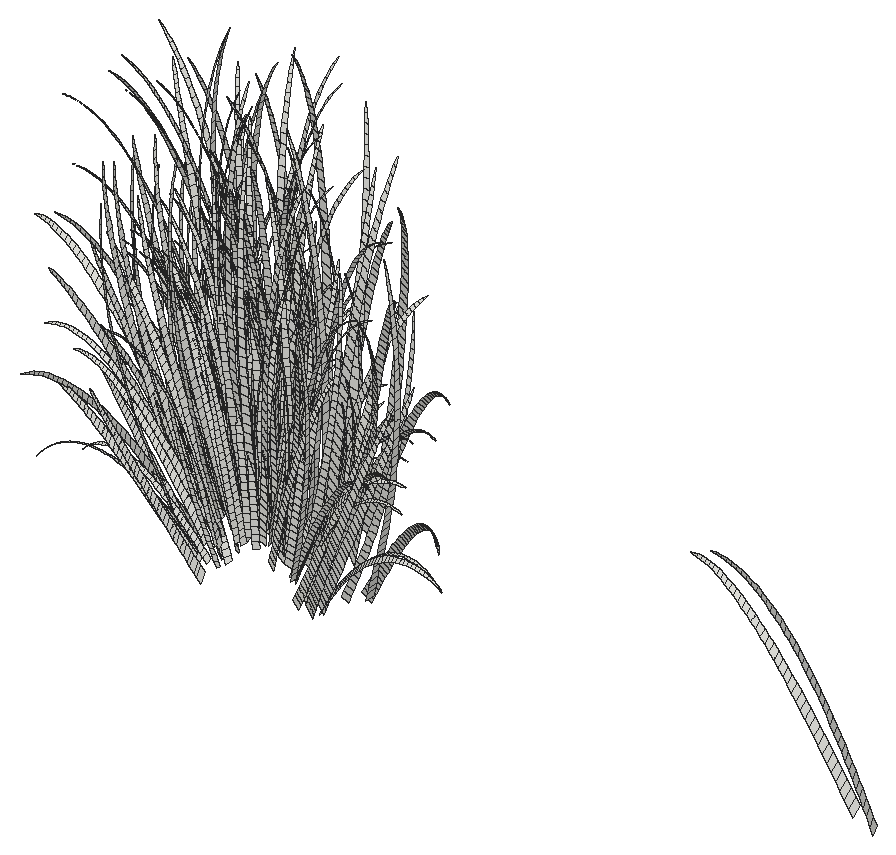
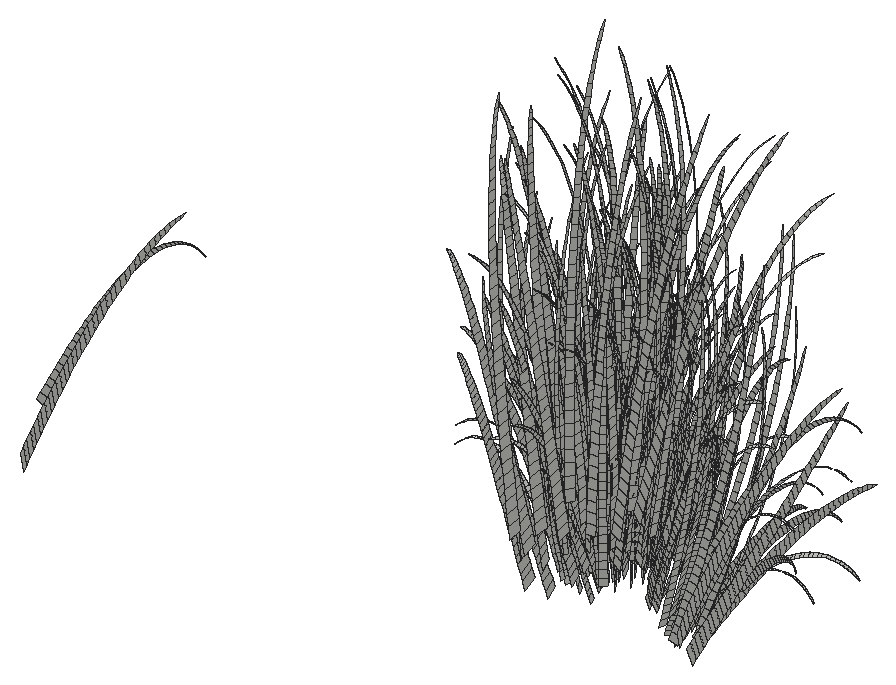
# SketchUp Ruby script. Lengths in inches.
U = 1.inch
M = Sketchup.active_model
def pt(a) = Geom::Point3d.new(a.map { |v| v * U })
def face(e, loops, mat)
  f = e.add_face(loops[0].map { |a| pt(a) })
  loops[1..].each { |l| e.add_face(l.map { |a| pt(a) }).erase! }
  f.material = f.back_material = mat if mat
  f
end
# faces: each face lists its corners as indices into pts; further lists are holes
def faces(e, pts, list, mat = nil) = list.each { |f| face(e, (f[0].is_a?(Array) ? f : [f]).map { |l| l.map { |i| pts[i] } }, mat) }
# xy, xz, yz: faces in a plane at the given z, y or x. An outline is a flat list of corners, or four numbers for a rectangle; further outlines are holes
def ring(l) = l.size == 4 ? [[l[0], l[1]], [l[2], l[1]], [l[2], l[3]], [l[0], l[3]]] : l.each_slice(2).to_a
def flat(e, list, mat, &to3) = list.each { |f| face(e, (f[0].is_a?(Array) ? f : [f]).map { |l| ring(l).map { |u, v| to3.(u, v) } }, mat) }
def xy(e, z, list, mat = nil) = flat(e, list, mat) { |x, y| [x, y, z] }
def xz(e, y, list, mat = nil) = flat(e, list, mat) { |x, z| [x, y, z] }
def yz(e, x, list, mat = nil) = flat(e, list, mat) { |y, z| [x, y, z] }
def lines(e, pts, list) = list.each { |a, b| e.add_line(pt(pts[a]), pt(pts[b])) }
# prism: a flat outline (further loops are holes) pulled along v
def prism(e, loops, v, mat = nil)
  f = face(e, loops, mat); d = Geom::Vector3d.new(v.map { |x| x * U })
  f.pushpull(f.normal.samedirection?(d) ? d.length : -d.length)
end
def box(e, o, s, mat = nil) = prism(e, [[o, [o[0] + s[0], o[1], o[2]], [o[0] + s[0], o[1] + s[1], o[2]], [o[0], o[1] + s[1], o[2]]]], [0, 0, s[2]], mat)
def at(x, y, z, deg = 0) = Geom::Transformation.translation(pt([x, y, z])) * Geom::Transformation.rotation(ORIGIN, Z_AXIS, deg.degrees)
def axes(o, x, y, z) = Geom::Transformation.new([*x, 0, *y, 0, *z, 0, *pt(o).to_a, 1])
def part(name) = M.definitions.add(name)
# library, detail: a bought-in or finely detailed component or shape, given as its bounding box
def library(name, o, s) = part(name).tap { |d| box(d.entities, o, s) }
def detail(e, o, s) = box(e.add_group.entities, o, s)
def put(e, d, t, mat = nil) = e.add_instance(d, t).tap { |i| i.material = mat if mat }
def group(e, t, mat = nil) = e.add_group.tap { |g| g.transformation = t; g.material = mat if mat }.entities
root = M.entities
c1 = part("fur_instance\#8")
p = [[-0.25,1.49,0.03],[0.25,-1.49,-0.03],[0.44,-1.47,1.51],[-0.05,1.47,1.57],[0.65,-1.44,3.05],[0.16,1.45,3.11],
  [0.86,-1.42,4.59],[0.38,1.44,4.65],[1.1,-1.39,6.13],[0.62,1.43,6.18],[1.34,-1.35,7.66],[0.875,1.42,7.72],
  [1.6,-1.32,9.19],[1.14,1.41,9.25],[1.88,-1.28,10.72],[1.43,1.41,10.78],[2.18,-1.24,12.25],[1.73,1.41,12.3],
  [2.49,-1.19,13.77],[2.05,1.41,13.82],[2.83,-1.15,15.29],[2.4,1.41,15.34],[3.18,-1.09,16.8],[2.76,1.42,16.85],
  [3.56,-1.03,18.31],[3.14,1.43,18.35],[3.96,-0.97,19.81],[3.55,1.44,19.85],[4.38,-0.91,21.3],[3.99,1.46,21.35],
  [4.84,-0.83,22.78],[4.45,1.48,22.83],[5.32,-0.76,24.26],[4.93,1.51,24.31],[5.82,-0.67,25.73],[5.45,1.54,25.77],
  [6.36,-0.59,27.18],[6,1.57,27.23],[6.93,-0.49,28.625],[6.58,1.61,28.67],[7.54,-0.39,30.05],[7.19,1.66,30.1],
  [8.18,-0.28,31.47],[7.84,1.71,31.51],[8.85,-0.16,32.86],[8.53,1.77,32.9],[9.57,-0.04,34.24],[9.25,1.83,34.27],
  [10.32,0.09,35.59],[10.02,1.9,35.625],[11.12,0.23,36.92],[10.82,1.97,36.95],[11.95,0.38,38.22],[11.67,2.06,38.25],
  [12.84,0.54,39.49],[12.57,2.14,39.52],[13.76,0.71,40.73],[13.51,2.24,40.76],[14.73,0.89,41.93],[14.49,2.34,41.95],
  [15.75,1.08,43.09],[15.52,2.45,43.11],[16.82,1.28,44.2],[16.6,2.5625,44.23],[17.93,1.5,45.27],[17.73,2.68,45.29],
  [19.08,1.73,46.28],[18.9,2.81,46.3],[20.29,1.97,47.24],[20.125,2.93,47.26],[21.53,2.22,48.13],[21.39,3.0625,48.15],
  [22.82,2.5,48.96],[22.7,3.1875,48.98],[24.14,2.8125,49.72],[24.06,3.3,49.73],[25.48,3.27,50.41]]
faces(c1.entities,p,[[0,1,2,3],[3,2,4,5],[5,4,6,7],[7,6,8,9],[9,8,10,11],[11,10,12,13],[13,12,14,15],[15,14,16,17],
  [17,16,18,19],[19,18,20,21],[21,20,22,23],[23,22,24,25],[25,24,26,27],[27,26,28,29],[29,28,30,31],[31,30,32,33],
  [33,32,34,35],[35,34,36,37],[37,36,38,39],[39,38,40,41],[41,40,42,43],[43,42,44,45],[45,44,46,47],[47,46,48,49],
  [49,48,50,51],[51,50,52,53],[53,52,54,55],[55,54,56,57],[57,56,58,59],[59,58,60,61],[61,60,62,63],[63,62,64,65],
  [65,64,66,67],[67,66,68,69],[69,68,70,71],[71,70,72,73],[73,72,74,75],[75,74,76]])
put(root,c1,axes([43.23,68.45,7.65],[-0.18691,0.1568,-0.23935],[-0.06787,-0.16218,-0.27405],[-0.15492,-0.08418,0.43132]))
put(root,c1,axes([42.47,71.27,4.78],[-0.09014,-0.18111,-0.08882],[0.15594,-0.13199,0.32093],[-0.15035,0.00199,0.40617]))
put(root,c1,axes([42.5,70.05,2.88],[0.01897,-0.21218,0.0586],[0.13531,-0.01729,0.38322],[-0.17657,-0.01268,0.31544]))
put(root,c1,axes([43.08,68.3125,3.14],[-0.03242,-0.16161,-0.19656],[0.13271,-0.12456,0.32589],[-0.17032,-0.04313,0.30667]))
put(root,c1,axes([44.46,67.32,5.39],[-0.17146,0.07712,-0.27655],[0.00216,-0.17859,-0.14821],[-0.13359,-0.07259,0.37194]))
put(root,c1,axes([44.12,67.44,2.26],[-0.07927,0.1771,-0.13212],[-0.09456,-0.05104,-0.31736],[-0.15384,-0.03896,0.27701]))
put(root,c1,axes([44.33,67.0625,3.02],[-0.11039,-0.00414,-0.3495],[0.07669,-0.1786,0.00651],[-0.14786,-0.06719,0.2791]))
put(root,c1,axes([44.91,65.8125,3.03],[-0.13594,0.15084,-0.11164],[-0.0609,-0.07291,-0.33491],[-0.13519,-0.09407,0.27953]))
put(root,c1,axes([42.62,69.58,3.24],[0.13391,-0.00422,0.37894],[-0.02725,0.21287,-0.08205],[-0.17659,-0.01268,0.31548]))
put(root,c1,axes([45.3,66.53,4.31],[-0.14992,0.10635,-0.20855],[-0.03569,-0.13875,-0.18978],[-0.12006,-0.06524,0.33426]))
put(root,c1,axes([45.29,67.96,4.18],[-0.13947,0.07457,-0.26376],[-0.03048,-0.16347,-0.05841],[-0.12421,-0.01975,0.3263]))
put(root,c1,axes([45.33,66.7,2.78],[-0.11214,0.07357,-0.29467],[-0.00419,-0.1506,-0.10442],[-0.13991,-0.03543,0.25192]))
put(root,c1,axes([44.39,70.26,10.76],[-0.16722,-0.14584,-0.14657],[0.18274,-0.19209,0.09427],[-0.0816,-0.06233,0.55718]))
put(root,c1,axes([42.92,71.21,4.29],[0.10956,-0.18152,0.25882],[0.13509,0.11782,0.19082],[-0.14519,0.00192,0.39222]))
put(root,c1,axes([43.91,69.17,3.66],[0.07012,-0.18381,0.20265],[0.10518,0.07075,0.29594],[-0.16336,-0.01173,0.29184]))
put(root,c1,axes([43.8,66.95,3.01],[0.11177,0.01694,0.37048],[-0.08915,0.18926,-0.03147],[-0.15727,-0.07147,0.29687]))
put(root,c1,axes([44.32,67.58,3.52],[0.07273,0.09595,0.27862],[-0.10249,0.16133,-0.212],[-0.15668,-0.03967,0.28211]))
put(root,c1,axes([42.84,68.47,4.28],[0.16226,-0.13696,0.26442],[0.06401,0.16282,0.19515],[-0.14822,-0.05035,0.39313]))
put(root,c1,axes([45.68,68.57,9.3],[-0.19486,-0.07064,-0.15993],[0.11436,-0.20339,0.01183],[-0.07048,-0.06892,0.50496]))
put(root,c1,axes([45.89,65.35,2.36],[-0.09839,0.14314,-0.01192],[-0.08354,-0.02419,-0.30566],[-0.11714,-0.08151,0.24221]))
put(root,c1,axes([45.28,68.2,2.86],[-0.01321,-0.17005,0.06481],[0.1141,-0.02557,0.30569],[-0.13946,0.01456,0.25678]))
put(root,c1,axes([46.39,69.16,7.12],[-0.18243,0.01895,-0.19563],[-0.00133,-0.1948,0.08688],[-0.09334,0.00298,0.40574]))
put(root,c1,axes([46.26,67.88,5.17],[-0.16023,0.03354,-0.19126],[-0.00898,-0.17162,0.02853],[-0.08895,-0.01176,0.36236]))
put(root,c1,axes([46.22,66.625,6.5],[-0.1494,0.14445,-0.05993],[-0.10862,-0.10225,-0.21391],[-0.08642,-0.08137,0.39881]))
put(root,c1,axes([43.7,68.125,5.17],[0.16036,-0.12824,0.26431],[0.05712,0.1633,0.18167],[-0.14465,-0.04914,0.38366]))
put(root,c1,axes([44.12,68.18,4.39],[0.12489,0.06673,0.27563],[-0.09958,0.18305,-0.12082],[-0.13573,-0.04611,0.36]))
put(root,c1,axes([46.51,66.73,5.01],[-0.15052,-0.00251,-0.18515],[0.03159,-0.16716,0.03488],[-0.08794,-0.02622,0.34898]))
put(root,c1,axes([46.24,68.69,5.72],[-0.10618,-0.13262,-0.04878],[0.13367,-0.1263,0.19427],[-0.08735,0.00279,0.37967]))
put(root,c1,axes([45.09,68.18,2.35],[0.10833,0.05099,0.24664],[-0.03776,0.16401,-0.19126],[-0.1393,0.01454,0.25647]))
put(root,c1,axes([46.21,70.78,11.94],[-0.09372,-0.20637,-0.07363],[0.22677,-0.12712,0.15354],[-0.08199,-0.04812,0.55353]))
put(root,c1,axes([44.63,69.19,4.82],[0.15491,-0.05585,0.29054],[0.02871,0.18789,-0.02061],[-0.13151,0.00174,0.35528]))
put(root,c1,axes([47.24,67.92,6.26],[-0.13836,0.10656,-0.19014],[-0.08729,-0.13946,-0.02631],[-0.08371,0.00267,0.36384]))
put(root,c1,axes([46.12,66.87,4.0625],[0.03066,0.14936,0.05869],[-0.12804,0.07175,-0.24213],[-0.11455,-0.01821,0.30092]))
put(root,c1,axes([46.49,66.9375,7.95],[-0.03053,0.18634,0.11663],[-0.19498,0.03215,-0.20672],[-0.09234,-0.08694,0.42611]))
put(root,c1,axes([46.73,66.09,6.54],[-0.076,0.1669,0.09562],[-0.17144,-0.01335,-0.19918],[-0.07397,-0.09509,0.39348]))
put(root,c1,axes([47.05,67.9,6.875],[-0.14595,-0.08896,-0.08701],[0.11069,-0.159,0.08949],[-0.05969,-0.02587,0.41282]))
put(root,c1,axes([47.0625,66.87,7.05],[-0.13003,0.1505,-0.04051],[-0.13515,-0.09639,-0.12681],[-0.0585,-0.05721,0.41915]))
put(root,c1,axes([47.05,69.73,10.85],[-0.20007,-0.1011,-0.05198],[0.13259,-0.20105,0.02025],[-0.03025,-0.05245,0.53866]))
put(root,c1,axes([47.55,69.61,11.96],[-0.23914,-0.05106,-0.06078],[0.08551,-0.22855,-0.0252],[-0.02809,-0.06875,0.5682]))
put(root,c1,axes([45.99,67.93,2.35],[0.06974,-0.11239,0.27242],[0.09117,0.10684,0.0892],[-0.12045,0.03482,0.23783]))
put(root,c1,axes([45.17,69.49,3.94],[0.12819,-0.10555,0.27193],[0.08655,0.15023,0.02614],[-0.11644,0.02211,0.33646]))
put(root,c1,axes([46.16,66.64,2.65],[0.09888,-0.02928,0.28041],[-0.00291,0.15131,-0.01175],[-0.12783,-0.00918,0.22836]))
put(root,c1,axes([46.68,68.41,4.28],[-0.01787,-0.16163,0.13786],[0.14541,-0.01364,0.20157],[-0.09392,0.03632,0.30351]))
put(root,c1,axes([47.6,66.9,6.07],[-0.15295,0.08658,-0.10984],[-0.06653,-0.14152,-0.02919],[-0.05435,-0.02356,0.3759]))
put(root,c1,axes([47.26,68.36,4.31],[-0.08732,-0.12975,0.07004],[0.12156,-0.08169,0.22443],[-0.07712,0.04857,0.29461]))
put(root,c1,axes([48.08,69.47,12.02],[-0.24023,0.10194,-0.01182],[-0.08393,-0.20819,-0.06775],[-0.02132,-0.07588,0.56748]))
put(root,c1,axes([45.8,66.95,4],[0.13512,-0.04534,0.25565],[0.00767,0.16418,0.01521],[-0.11775,-0.01872,0.30933]))
put(root,c1,axes([47.95,66.88,6.03],[-0.16155,0.04363,-0.11105],[-0.02173,-0.15615,0.00187],[-0.05311,-0.02302,0.36735]))
put(root,c1,axes([47.87,68.14,5.93],[-0.13763,-0.08778,-0.02445],[0.09224,-0.14199,0.18002],[-0.06167,0.02548,0.35158]))
put(root,c1,axes([47.56,67.91,10.37],[-0.11071,0.19643,0.08485],[-0.20741,-0.05916,-0.14436],[-0.04649,-0.10158,0.50968]))
put(root,c1,axes([45.88,67.375,6.29],[0.12398,0.09622,0.18511],[-0.12468,0.16008,-0.11198],[-0.09878,-0.04719,0.39625]))
put(root,c1,axes([48.19,67.29,6.85],[-0.15275,-0.06369,-0.07605],[0.08272,-0.1606,0.08732],[-0.05298,-0.01559,0.38969]))
put(root,c1,axes([48.03,66.44,6.02],[-0.12167,0.12231,-0.08026],[-0.10576,-0.10199,-0.07795],[-0.05387,-0.03162,0.36369]))
put(root,c1,axes([46.53,67.73,6.44],[0.1073,0.11537,0.13468],[-0.12896,0.14123,-0.15523],[-0.09593,-0.0286,0.38067]))
put(root,c1,axes([48.43,66.98,5.86],[-0.15222,0.06371,-0.10078],[-0.04912,-0.14483,0.02613],[-0.04368,-0.00705,0.35627]))
put(root,c1,axes([48.58,66.57,7.68],[-0.18454,0.07316,-0.01839],[-0.05778,-0.16138,-0.04792],[-0.01906,-0.05522,0.43193]))
put(root,c1,axes([47.28,71.5625,10.61],[-0.03022,-0.22611,0.09029],[0.23429,-0.05028,0.11994],[-0.05481,-0.00145,0.5217]))
put(root,c1,axes([46.77,65.9,6.75],[0.08886,0.11953,0.22309],[-0.17307,0.12603,-0.0526],[-0.07674,-0.09865,0.40821]))
put(root,c1,axes([48.6875,69.69,11.16],[-0.19122,-0.11806,-0.01455],[0.14538,-0.19433,0.04316],[-0.02276,-0.03764,0.53822]))
put(root,c1,axes([47.69,68.76,7.33],[-0.07059,-0.16734,0.04684],[0.17777,-0.08469,0.11217],[-0.04438,-0.00118,0.42241]))
put(root,c1,axes([48.78,67.4,6.72],[-0.1632,-0.04584,-0.02491],[0.06111,-0.16287,0.10545],[-0.03205,0.00396,0.38155]))
put(root,c1,axes([48.01,67.78,6.35],[-0.07809,-0.14325,0.0107],[0.15359,-0.09235,0.11164],[-0.04706,-0.00759,0.38378]))
put(root,c1,axes([48.86,68.24,7.62],[-0.18597,0.0618,-0.02273],[-0.04748,-0.17087,0.02426],[-0.01189,-0.02692,0.4292]))
put(root,c1,axes([47.125,67.35,3.82],[0.12505,0.02128,0.17693],[-0.02026,0.14885,-0.13694],[-0.09536,0.01811,0.27556]))
put(root,c1,axes([45.24,70.37,10.84],[0.23978,-0.07082,0.15768],[0.03022,0.22441,0.06362],[-0.07961,-0.06081,0.54364]))
put(root,c1,axes([47.99,68.31,8.97],[-0.04674,0.1979,-0.00041],[-0.20698,-0.02041,-0.04932],[-0.02674,-0.04637,0.47621]))
put(root,c1,axes([45.64,68.09,10.33],[0.21026,0.07749,0.17035],[-0.13208,0.20951,0.0486],[-0.06062,-0.09852,0.54406]))
put(root,c1,axes([46,69.1,8.38],[0.19711,0.03834,0.13931],[-0.07116,0.20343,-0.04176],[-0.07003,-0.0411,0.47276]))
put(root,c1,axes([47.35,67.91,5.18],[0.08378,-0.14307,0.16626],[0.13275,0.07958,0.06416],[-0.07048,0.0146,0.34149]))
put(root,c1,axes([49.15,65.47,5.87],[-0.14611,0.07417,-0.01085],[-0.0636,-0.12579,-0.04088],[-0.01571,-0.04551,0.35595]))
put(root,c1,axes([48.66,65.52,5.8125],[-0.03907,0.14419,0.04289],[-0.15068,-0.00691,-0.10234],[-0.04404,-0.05511,0.34471]))
put(root,c1,axes([49.46,66.39,7.91],[-0.18895,0.06999,0.02245],[-0.05996,-0.16418,-0.04942],[-0.00199,-0.06326,0.44045]))
put(root,c1,axes([48.5,68.33,10.35],[-0.07149,0.20688,0.05021],[-0.22153,-0.04139,-0.03916],[-0.01557,-0.07173,0.51835]))
put(root,c1,axes([49.1,67.78,4.94],[-0.12985,-0.07677,0.07158],[0.09092,-0.12597,0.14453],[-0.01646,0.03757,0.31821]))
put(root,c1,axes([48.59,66.36,6.02],[0.0007,0.15498,-0.03624],[-0.15701,0.01919,-0.0982],[-0.04789,-0.01409,0.35225]))
put(root,c1,axes([46.38,69.85,9.25],[0.21533,-0.00022,0.14201],[-0.02985,0.21622,-0.04212],[-0.07083,-0.0307,0.48991]))
put(root,c1,axes([48.5,69.9,7.23],[-0.05762,-0.17661,0.09378],[0.18885,-0.07013,0.07584],[-0.02585,0.00825,0.42914]))
put(root,c1,axes([49.21,66.12,7.21],[-0.11204,0.14362,0.03398],[-0.14775,-0.08605,-0.03808],[-0.00899,-0.05843,0.41243]))
put(root,c1,axes([48.16,66.88,6.26],[0.07256,0.13813,0.01061],[-0.14853,0.08916,-0.10968],[-0.05042,-0.01484,0.37084]))
put(root,c1,axes([50.02,68.28,8.42],[-0.20122,0.04978,0.02765],[-0.03696,-0.18587,0.02525],[0.00919,-0.0352,0.4569]))
put(root,c1,axes([48.82,69.16,8.53],[-0.07053,-0.17965,0.10788],[0.19435,-0.08267,0.06265],[-0.01549,0.01046,0.44704]))
put(root,c1,axes([49.43,67,6],[-0.12044,0.11617,-0.06507],[-0.11184,-0.10532,0.07409],[-0.00291,0.00808,0.35453]))
put(root,c1,axes([47.83,66.82,7.39],[0.1306,0.09776,0.12408],[-0.13059,0.14634,-0.04229],[-0.05761,-0.05634,0.41276]))
put(root,c1,axes([49.6875,67,6.24],[-0.14146,0.09732,-0.03277],[-0.08974,-0.12702,0.09515],[0.00654,0.00629,0.36155]))
put(root,c1,axes([49,66.14,7.75],[-0.02865,0.1632,0.13083],[-0.19416,0.00105,-0.04665],[-0.01776,-0.09378,0.4187]))
put(root,c1,axes([46.95,68.21,9.875],[0.21896,0.00722,0.14738],[-0.05367,0.20894,0.06409],[-0.06377,-0.07981,0.49923]))
put(root,c1,axes([48.88,66.79,6.33],[-0.005,0.15882,-0.01867],[-0.16818,0.01184,-0.02587],[-0.01594,-0.02637,0.37698]))
put(root,c1,axes([49.86,68.37,4.63],[-0.15178,-0.03817,0.09021],[0.05761,-0.14672,0.13772],[0.01323,0.03497,0.32535]))
put(root,c1,axes([49.83,68.04,5.2],[-0.14817,-0.05096,0.10268],[0.07099,-0.14472,0.13123],[0.01339,0.03539,0.32926]))
put(root,c1,axes([49.39,65.7,6.36],[-0.04364,0.1509,0.04181],[-0.16335,-0.02313,-0.02043],[-0.0082,-0.05328,0.37608]))
put(root,c1,axes([47.99,66.81,7.1],[0.16328,0.03799,0.12354],[-0.06943,0.16853,-0.0179],[-0.05845,-0.04464,0.39911]))
put(root,c1,axes([49.58,68.17,6.03],[-0.0829,-0.13844,0.09301],[0.15279,-0.09132,0.04718],[-0.00308,0.00854,0.37496]))
put(root,c1,axes([48.125,68.7,7.37],[0.11915,-0.15444,0.11959],[0.14734,0.10329,0.01409],[-0.04397,-0.00116,0.41847]))
put(root,c1,axes([47.6,68.36,7],[0.18469,-0.02182,0.1026],[0.00322,0.18141,-0.06268],[-0.05045,-0.00814,0.41143]))
put(root,c1,axes([49.71,67.02,9.15],[-0.06667,0.19226,0.05915],[-0.20819,-0.04319,-0.00198],[0.00188,-0.06909,0.48578]))
put(root,c1,axes([49.83,68.83,6.88],[-0.10911,-0.1372,0.1051],[0.15387,-0.1168,0.04236],[0.00736,0.00708,0.40712]))
put(root,c1,axes([48.25,66.2,5.88],[0.15146,0.01629,0.10652],[-0.04117,0.15418,-0.02273],[-0.05245,-0.03078,0.35407]))
put(root,c1,axes([48.97,69.19,7.38],[0.00836,-0.18662,0.11674],[0.19508,-0.00753,0.01588],[-0.01463,0.00988,0.4222]))
put(root,c1,axes([47.9375,68.6,8.75],[0.12224,-0.1724,0.03147],[0.17004,0.09672,0.03094],[-0.02457,-0.03858,0.46994]))
put(root,c1,axes([49.16,71.77,10.15],[-0.01914,-0.22341,0.14227],[0.23668,-0.03758,0.00754],[-0.0042,0.01167,0.5122]))
put(root,c1,axes([50.11,65.51,5.88],[-0.08483,0.12977,0.03637],[-0.13576,-0.06868,0.01436],[0.01015,-0.0438,0.35695]))
put(root,c1,axes([50.26,67.86,8.11],[-0.11995,-0.14094,0.03187],[0.15995,-0.12378,-0.02155],[0.01135,-0.03745,0.44662]))
put(root,c1,axes([48.36,66.92,7.55],[0.13112,0.1119,0.04642],[-0.13781,0.13647,-0.01148],[-0.02271,-0.04835,0.42618]))
put(root,c1,axes([47.47,67.25,9.9],[0.22597,0.02863,0.10796],[-0.07525,0.20019,0.13019],[-0.03474,-0.10937,0.51158]))
put(root,c1,axes([50.32,70.6,8.12],[-0.12335,-0.15584,0.12717],[0.17408,-0.13265,0.02266],[0.01997,0.00343,0.46197]))
put(root,c1,axes([49.59,68.51,8.48],[-0.03248,-0.18789,0.03246],[0.20264,-0.04691,-0.01246],[0.00277,-0.0305,0.45814]))
put(root,c1,axes([48.99,70.71,6.02],[0.06236,-0.17527,0.19539],[0.18475,0.04701,-0.03446],[-0.02024,0.04621,0.39144]))
put(root,c1,axes([47.11,70.18,11.9375],[0.24246,-0.09581,0.04741],[0.07374,0.21618,0.03906],[-0.03158,-0.05994,0.56838]))
put(root,c1,axes([49.34,69.22,8.65],[0.00458,-0.19714,0.03462],[0.20895,-0.01368,-0.00104],[-0.00501,-0.02872,0.46671]))
put(root,c1,axes([48.8,66.2,9.51],[0.08928,0.17665,0.16183],[-0.22737,0.09539,0.05927],[-0.00818,-0.11915,0.51927]))
put(root,c1,axes([48.28,68.33,6.17],[0.167,0.03821,0.03014],[-0.05354,0.16593,-0.1048],[-0.03226,0.00399,0.38398]))
put(root,c1,axes([50.59,67.23,5.52],[-0.11227,0.12169,-0.01571],[-0.11695,-0.0983,0.09825],[0.0234,-0.00238,0.35291]))
put(root,c1,axes([50.0625,68.5,11.01],[-0.01737,0.2214,0.05487],[-0.24332,0.00145,0.03189],[0.01003,-0.07326,0.54284]))
put(root,c1,axes([49.8125,65.79,7.98],[-0.01068,0.1751,0.14296],[-0.21108,0.00073,0.04004],[0.01667,-0.10172,0.45077]))
put(root,c1,axes([50.29,68.3,8.69],[-0.03706,0.19452,0.0025],[-0.2058,-0.02021,0.04233],[0.01369,-0.04269,0.4672]))
put(root,c1,axes([49.82,67.62,8.68],[0.00321,0.19067,0.02092],[-0.20749,0.01649,0.04397],[0.01444,-0.0534,0.46311]))
put(root,c1,axes([49.66,66.97,6.57],[0.0444,0.15353,-0.02873],[-0.16709,0.05572,0.00025],[-0.00083,-0.02443,0.38596]))
put(root,c1,axes([48.28,67.77,7.97],[0.19137,0.02245,0.03812],[-0.04546,0.1843,-0.01629],[-0.02307,-0.03624,0.44138]))
put(root,c1,axes([49.3125,69.2,9.86],[0.0752,-0.20516,0.02464],[0.21175,0.0536,-0.02901],[0.00304,-0.03339,0.50163]))
put(root,c1,axes([49.13,70.36,5.9],[0.1059,-0.15637,0.15831],[0.16025,0.08485,-0.11228],[-0.00207,0.04487,0.3837]))
put(root,c1,axes([51.53,69.14,10.47],[-0.20879,-0.09834,0.1321],[0.10662,-0.20129,-0.08744],[0.06463,-0.06137,0.52082]))
put(root,c1,axes([49.85,67.43,6.51],[0.04623,0.15623,-0.10375],[-0.16763,0.05842,0.01792],[0.01628,0.0028,0.37652]))
put(root,c1,axes([49.13,66.62,6.39],[0.15712,0.04243,0.01115],[-0.06087,0.1538,-0.0283],[-0.01337,-0.02475,0.37716]))
put(root,c1,axes([50.33,67.09,5.96],[-0.02615,-0.15514,0.08978],[0.1636,-0.03862,-0.04775],[0.02391,-0.00243,0.36067]))
put(root,c1,axes([49.03,68.37,5.91],[0.17226,-0.02677,0.04434],[0.01787,0.15893,-0.17055],[-0.01798,0.04104,0.34767]))
put(root,c1,axes([48.93,69.57,8.41],[0.17834,-0.11625,0.08266],[0.1071,0.16149,-0.09447],[-0.01558,0.01053,0.44981]))
put(root,c1,axes([51.7,67.0625,7.54],[-0.15292,0.11854,0.12624],[-0.12574,-0.14279,0.04956],[0.05301,-0.06232,0.4383]))
put(root,c1,axes([50.94,68.91,5.47],[-0.09023,-0.13424,0.18354],[0.14991,-0.10591,-0.00994],[0.04513,0.02354,0.36032]))
put(root,c1,axes([50.5,66.69,5.875],[0.01188,0.15545,-0.07184],[-0.16156,0.0237,0.07132],[0.03067,-0.00873,0.35494]))
put(root,c1,axes([50.4375,65.76,6.29],[-0.00201,0.1516,0.05729],[-0.16575,-0.0022,0.09935],[0.04109,-0.06021,0.3647]))
put(root,c1,axes([51.83,67.33,4.875],[-0.15312,0.05179,0.12153],[-0.03636,-0.15379,0.12597],[0.06399,-0.0008,0.33763]))
put(root,c1,axes([49.85,66.54,6.17],[0.13491,0.07893,-0.02845],[-0.09527,0.13412,-0.00523],[0.005,-0.02625,0.36875]))
put(root,c1,axes([50.57,69.04,5.39],[0.00974,-0.16765,0.16266],[0.17627,-0.01134,-0.08044],[0.03031,0.03221,0.35757]))
put(root,c1,axes([51.41,66.65,5.55],[-0.12808,-0.08127,0.17105],[0.08472,-0.13879,-0.03962],[0.07069,-0.01437,0.33524]))
put(root,c1,axes([50.51,72.16,12.29],[-0.01557,-0.2472,0.11257],[0.25666,-0.03446,-0.11464],[0.04868,-0.01385,0.56337]))
put(root,c1,axes([49.74,68.8,11.75],[0.1638,0.16225,0.02835],[-0.19372,0.16204,0.06129],[0.00656,-0.07857,0.56406]))
put(root,c1,axes([50.24,67.81,4.79],[0.06075,-0.14439,0.11282],[0.14535,0.04045,-0.11615],[0.02704,0.02874,0.31908]))
put(root,c1,axes([50.65,67.84,9.59],[0.00546,0.20018,0.07075],[-0.21886,0.00452,0.13393],[0.05427,-0.07952,0.48166]))
put(root,c1,axes([49.7,69.05,9.45],[0.1489,-0.1631,0.00196],[0.16131,0.12724,-0.0384],[0.00665,-0.0349,0.49014]))
put(root,c1,axes([52.26,68.03,6.35],[-0.17727,-0.00884,0.19718],[0.01815,-0.18643,0.05134],[0.08203,-0.01667,0.38902]))
put(root,c1,axes([49.21,68.81,10.99],[0.24085,-0.01288,-0.01594],[-0.00713,0.21681,0.06326],[0.00207,-0.07616,0.53545]))
put(root,c1,axes([52.34,68.4,7.99],[-0.19467,0.01004,0.22404],[-0.00781,-0.20399,0.04036],[0.09618,-0.03688,0.42982]))
put(root,c1,axes([49.22,69.48,12.1],[0.24462,0.04853,-0.00958],[-0.07419,0.22591,0.06737],[0.00661,-0.07917,0.56836]))
put(root,c1,axes([49.98,67.41,6.29],[0.16085,-0.07091,-0.00868],[0.05991,0.14859,-0.10356],[0.01607,0.00276,0.37166]))
put(root,c1,axes([51.96,66.49,4.85],[-0.09933,0.11915,0.09682],[-0.11277,-0.10305,0.14649],[0.07419,-0.02845,0.33155]))
put(root,c1,axes([50.7,65.87,8.07],[0.1142,0.15271,0.07486],[-0.18421,0.10064,0.13224],[0.02836,-0.10071,0.46512]))
put(root,c1,axes([51.125,66.91,4.8],[0.01848,-0.15029,0.09797],[0.14831,0.00119,-0.12824],[0.05045,0.01072,0.31409]))
put(root,c1,axes([49.84,67.96,9.53],[0.21441,0.03504,-0.02755],[-0.05444,0.19871,0.04867],[0.01191,-0.06374,0.49276]))
put(root,c1,axes([50.35,66.59,5.8],[0.15483,0.02452,-0.08835],[-0.03742,0.15266,-0.04583],[0.03016,-0.00858,0.34899]))
put(root,c1,axes([50.84,66.39,5.48],[0.12172,0.08749,-0.09823],[-0.09805,0.12464,0.01693],[0.03543,-0.01566,0.34464]))
put(root,c1,axes([52.38,70.26,7.03],[-0.10531,-0.16415,0.20039],[0.16955,-0.12413,-0.09552],[0.08116,-0.00102,0.4282]))
put(root,c1,axes([50.39,67.3,7.19],[0.15584,0.0797,-0.11547],[-0.0923,0.15744,0.00315],[0.04105,-0.01815,0.39937]))
put(root,c1,axes([53.4375,68.26,8.11],[-0.20296,0.04396,0.25147],[-0.06114,-0.20583,-0.00189],[0.10319,-0.08007,0.46398]))
put(root,c1,axes([52.16,66.9,5.95],[-0.05241,0.16147,0.07727],[-0.15892,-0.06034,0.18232],[0.08415,-0.0479,0.3696]))
put(root,c1,axes([51.12,66.85,6.45],[0.10935,0.12723,-0.0806],[-0.13524,0.11022,0.08276],[0.04716,-0.03593,0.38648]))
put(root,c1,axes([52.63,66.15,4.19],[-0.13363,0.01209,0.24348],[-0.02341,-0.15821,0.02454],[0.10585,-0.04288,0.29749]))
put(root,c1,axes([51.33,65.54,5.03],[0.04868,0.13833,-0.04452],[-0.13249,0.04478,0.16098],[0.07098,-0.0404,0.31175]))
put(root,c1,axes([50.79,68.62,4.46],[0.15705,-0.06817,-0.01855],[0.04537,0.13415,-0.23216],[0.04015,0.05663,0.29621]))
put(root,c1,axes([51.9,66.96,4.26],[-0.0035,0.15221,-0.13037],[-0.13811,0.0204,0.18439],[0.08356,0.01425,0.28222]))
put(root,c1,axes([50.85,68.01,10.22],[0.18476,0.1259,-0.03463],[-0.14125,0.16417,0.15823],[0.05053,-0.09421,0.50755]))
put(root,c1,axes([52.91,67.04,5.07],[-0.105,0.10997,0.20265],[-0.1047,-0.1341,0.17455],[0.11569,-0.04687,0.32514]))
put(root,c1,axes([51.11,68.72,7.45],[0.18917,-0.06704,-0.06686],[0.05451,0.17895,-0.10326],[0.03727,-0.0106,0.43133]))
put(root,c1,axes([52.45,67.5,2.3],[-0.02967,-0.12807,0.22483],[0.11753,-0.07372,-0.14887],[0.10049,0.02798,0.22698]))
put(root,c1,axes([50.7,69.07,9.47],[0.21551,0.00607,-0.13742],[-0.0172,0.21045,-0.03067],[0.05502,-0.03283,0.47913]))
put(root,c1,axes([51.1875,67.71,7.47],[0.18544,-0.04972,-0.1199],[0.04511,0.1779,-0.04118],[0.05175,-0.03943,0.42412]))
put(root,c1,axes([54.02,69.2,8.55],[-0.13857,0.17143,0.18015],[-0.17196,-0.14956,0.18932],[0.11106,-0.06322,0.48777]))
put(root,c1,axes([53.35,69.35,4.41],[-0.08271,-0.14836,0.25336],[0.14839,-0.11682,-0.11362],[0.10275,0.01753,0.34702]))
put(root,c1,axes([51.64,67.73,4.09],[0.1392,0.01865,-0.19659],[-0.04604,0.15192,-0.11441],[0.07206,0.03039,0.28637]))
put(root,c1,axes([51.29,69.6875,9.46],[0.2045,-0.09371,-0.11076],[0.08595,0.19464,-0.09275],[0.05645,-0.03369,0.4916]))
put(root,c1,axes([51.76,71.22,8.87],[0.13505,-0.18869,0.02697],[0.17317,0.11473,-0.23558],[0.07413,0.01575,0.4615]))
put(root,c1,axes([53.84,68.18,7.42],[-0.05009,0.1972,0.12811],[-0.20341,-0.06615,0.21296],[0.10198,-0.07913,0.45854]))
put(root,c1,axes([53.43,67.67,4.72],[-0.05226,0.17384,0.04608],[-0.14605,-0.06174,0.27189],[0.11826,-0.02606,0.33853]))
put(root,c1,axes([52.99,65.9375,2.64],[-0.0259,0.13847,0.08839],[-0.10293,-0.05886,0.26708],[0.12297,-0.03787,0.2304]))
put(root,c1,axes([51.89,67.41,7.26],[0.19428,0.00099,-0.13011],[-0.00447,0.1857,0.01775],[0.05358,-0.05088,0.43173]))
put(root,c1,axes([53.22,67.67,2.89],[-0.0586,-0.13145,0.25194],[0.10919,-0.10295,-0.16429],[0.12358,0.00811,0.25105]))
put(root,c1,axes([52.13,66.77,3.86],[0.11365,-0.08796,-0.13302],[0.06535,0.12495,-0.18142],[0.09174,-0.00314,0.27875]))
put(root,c1,axes([52.65,68.98,4.39],[0.12182,-0.13641,-0.05722],[0.10481,0.11532,-0.25636],[0.0972,0.01658,0.32827]))
put(root,c1,axes([52.4,68.15,4.98],[0.15112,-0.07348,-0.15621],[0.04279,0.15836,-0.20373],[0.095,0.01621,0.32084]))
put(root,c1,axes([54.1,67.97,8.33],[0.03711,0.21617,0.09276],[-0.22705,0.0107,0.25479],[0.10293,-0.10542,0.49477]))
put(root,c1,axes([53.39,68.18,6.59],[0.10459,0.17012,-0.10766],[-0.16118,0.10117,0.20027],[0.09662,-0.055,0.42437]))
put(root,c1,axes([54.92,68.55,2.53],[-0.11534,0.10838,0.24896],[-0.07338,-0.1624,0.25205],[0.15325,-0.01897,0.29298]))
put(root,c1,axes([52.91,66.17,4.37],[0.13705,0.06092,-0.24143],[-0.03897,0.15511,0.08813],[0.11117,-0.04504,0.31244]))
put(root,c1,axes([54.62,69.52,5.1],[-0.04683,-0.20253,0.13494],[0.1704,-0.05617,-0.28372],[0.13472,-0.02969,0.38568]))
put(root,c1,axes([53.18,66.62,3.78],[0.14053,0.00256,-0.25431],[0.0115,0.16488,-0.00221],[0.11001,-0.04457,0.30917]))
put(root,c1,axes([53.41,67.55,4.1],[0.11573,-0.11352,-0.17299],[0.09518,0.13737,-0.20258],[0.11423,-0.02517,0.32701]))
put(root,c1,axes([54.25,65.75,2.62],[0.04443,0.16095,0.1082],[-0.13761,-0.02397,0.33152],[0.13789,-0.09974,0.2801]))
put(root,c1,axes([54.78,72.45,8.49],[0.03522,-0.24577,0.05534],[0.23308,0.0235,-0.26379],[0.10852,-0.02206,0.51462]))
put(root,c1,axes([54.58,66.45,2.75],[0.00679,0.17207,0.10989],[-0.13694,-0.04896,0.33579],[0.14998,-0.07528,0.28652]))
put(root,c1,axes([54.29,70.35,7.98],[0.1074,-0.20139,-0.09354],[0.19115,0.11076,-0.2385],[0.10824,-0.04151,0.48371]))
put(root,c1,axes([53.65,69.12,5.15],[0.15027,-0.10781,-0.18095],[0.0791,0.16599,-0.22838],[0.11882,-0.00407,0.36105]))
put(root,c1,axes([56.84,68.63,3.29],[-0.15284,0.01805,0.42901],[-0.06641,-0.2167,0.01891],[0.18229,-0.0915,0.34824]))
put(root,c1,axes([54.53,67.28,2.8],[0.12633,-0.01434,-0.33979],[0.03003,0.18353,-0.05493],[0.15045,-0.04633,0.28189]))
put(root,c1,axes([54.75,66.42,2.67],[0.13942,0.04831,-0.34302],[0.00816,0.17572,0.1089],[0.15278,-0.07668,0.29185]))
put(root,c1,axes([55,70.61,6.52],[0.12813,-0.17071,-0.17976],[0.14324,0.15198,-0.29056],[0.14651,-0.03228,0.41943]))
put(root,c1,axes([56.27,69.0625,2.92],[0.07286,-0.17069,-0.21842],[0.13329,0.1313,-0.33824],[0.176,-0.05419,0.32974]))
put(root,c1,axes([96.49,68.45,1.73],[-0.18691,0.1568,-0.23935],[-0.06787,-0.16218,-0.27405],[-0.15492,-0.08418,0.43132]))
put(root,c1,axes([95.73,71.27,-1.14],[-0.09014,-0.18111,-0.08882],[0.15594,-0.13199,0.32093],[-0.15035,0.00199,0.40617]))
